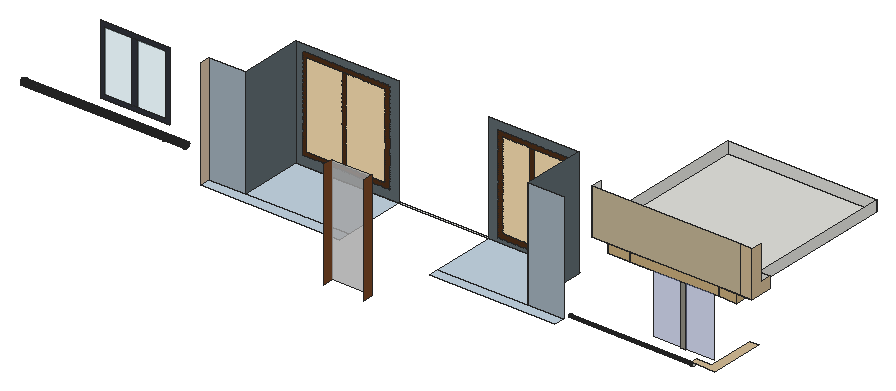
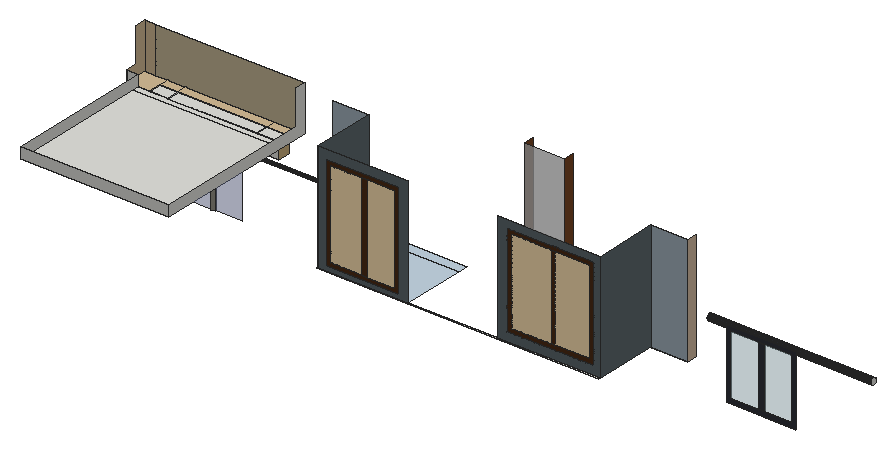
# SketchUp Ruby script. Lengths in inches.
U = 1.inch
M = Sketchup.active_model
def pt(a) = Geom::Point3d.new(a.map { |v| v * U })
def face(e, loops, mat)
  f = e.add_face(loops[0].map { |a| pt(a) })
  loops[1..].each { |l| e.add_face(l.map { |a| pt(a) }).erase! }
  f.material = f.back_material = mat if mat
  f
end
# faces: each face lists its corners as indices into pts; further lists are holes
def faces(e, pts, list, mat = nil) = list.each { |f| face(e, (f[0].is_a?(Array) ? f : [f]).map { |l| l.map { |i| pts[i] } }, mat) }
# xy, xz, yz: faces in a plane at the given z, y or x. An outline is a flat list of corners, or four numbers for a rectangle; further outlines are holes
def ring(l) = l.size == 4 ? [[l[0], l[1]], [l[2], l[1]], [l[2], l[3]], [l[0], l[3]]] : l.each_slice(2).to_a
def flat(e, list, mat, &to3) = list.each { |f| face(e, (f[0].is_a?(Array) ? f : [f]).map { |l| ring(l).map { |u, v| to3.(u, v) } }, mat) }
def xy(e, z, list, mat = nil) = flat(e, list, mat) { |x, y| [x, y, z] }
def xz(e, y, list, mat = nil) = flat(e, list, mat) { |x, z| [x, y, z] }
def yz(e, x, list, mat = nil) = flat(e, list, mat) { |y, z| [x, y, z] }
def lines(e, pts, list) = list.each { |a, b| e.add_line(pt(pts[a]), pt(pts[b])) }
# prism: a flat outline (further loops are holes) pulled along v
def prism(e, loops, v, mat = nil)
  f = face(e, loops, mat); d = Geom::Vector3d.new(v.map { |x| x * U })
  f.pushpull(f.normal.samedirection?(d) ? d.length : -d.length)
end
def box(e, o, s, mat = nil) = prism(e, [[o, [o[0] + s[0], o[1], o[2]], [o[0] + s[0], o[1] + s[1], o[2]], [o[0], o[1] + s[1], o[2]]]], [0, 0, s[2]], mat)
def at(x, y, z, deg = 0) = Geom::Transformation.translation(pt([x, y, z])) * Geom::Transformation.rotation(ORIGIN, Z_AXIS, deg.degrees)
def axes(o, x, y, z) = Geom::Transformation.new([*x, 0, *y, 0, *z, 0, *pt(o).to_a, 1])
def part(name) = M.definitions.add(name)
# library, detail: a bought-in or finely detailed component or shape, given as its bounding box
def library(name, o, s) = part(name).tap { |d| box(d.entities, o, s) }
def detail(e, o, s) = box(e.add_group.entities, o, s)
def put(e, d, t, mat = nil) = e.add_instance(d, t).tap { |i| i.material = mat if mat }
def group(e, t, mat = nil) = e.add_group.tap { |g| g.transformation = t; g.material = mat if mat }.entities
root = M.entities
M.materials.add("[0032_Moccasin]").color = [255, 228, 181]
M.materials.add("[Formica Beige]").color = [211, 187, 149]
M.materials.add("[Formica Graystone]").color = [149, 146, 135]
M.materials.add("[Formica Laminate Dark]").color = [50, 53, 60]
M.materials.add("[Formica Laminate Light]").color = [213, 189, 164]
M.materials.add("[Formica Speckled Grey]").color = [94, 105, 111]
M.materials.add("[Quartz Light Brown]").color = [199, 184, 152]
M.materials.add("[Terrazzo Light Blue]1").color = [165, 180, 191]
M.materials.add("[Terrazzo Light Blue]2").color = [196, 214, 227]
M.materials.add("[Translucent Glass Safety]").color = [204, 235, 244]
M.materials["[Translucent Glass Safety]"].alpha = 0.5
M.materials.add("[Translucent Glass Sky Reflection]").color = [126, 138, 183]
M.materials["[Translucent Glass Sky Reflection]"].alpha = 0.52
M.materials.add("[Translucent Resin Crush Gray]").color = [201, 201, 201]
M.materials["[Translucent Resin Crush Gray]"].alpha = 0.8
M.materials.add("[Wood Floor Light]").color = [204, 176, 127]
M.materials.add("[Wood Veneer 01]").color = [79, 46, 24]
M.materials.add("[Wood Veneer 01]2").color = [120, 70, 37]
xy(root,525,[[238.58,216.84,549.2,218.65]])
xy(root,525,[[198.57,135.71,351.88,147.05],[450.54,135.71,588.3,147.05],[238.58,147.05,351.88,216.84],[450.54,147.05,549.2,216.84]],"[Terrazzo Light Blue]2")
xy(root,544.8125,[[666.73,124.73,667.14,124.78,667.51,124.94,667.84,125.1875,668.09,125.51,668.24,125.89,668.3,126.29,668.24,126.7,668.09,127.07,667.84,127.4,667.51,127.65,667.14,127.8,666.73,127.86,666.33,127.8,665.95,127.65,665.63,127.4,665.38,127.07,665.22,126.7,665.17,126.29,665.22,125.89,665.38,125.51,665.63,125.1875,665.95,124.94,666.33,124.78],[693.42,124.73,693.83,124.78,694.2,124.94,694.53,125.1875,694.77,125.51,694.93,125.89,694.98,126.29,694.93,126.7,694.77,127.07,694.53,127.4,694.2,127.65,693.83,127.8,693.42,127.86,693.02,127.8,692.64,127.65,692.32,127.4,692.07,127.07,691.91,126.7,691.86,126.29,691.91,125.89,692.07,125.51,692.32,125.1875,692.64,124.94,693.02,124.78],[709.48,124.73,709.89,124.78,710.26,124.94,710.59,125.1875,710.84,125.51,710.99,125.89,711.05,126.29,710.99,126.7,710.84,127.07,710.59,127.4,710.26,127.65,709.89,127.8,709.48,127.86,709.08,127.8,708.7,127.65,708.38,127.4,708.13,127.07,707.97,126.7,707.92,126.29,707.97,125.89,708.13,125.51,708.38,125.1875,708.7,124.94,709.08,124.78]])
xy(root,545.4375,[[621.3,124.73,621.7,124.78,622.08,124.94,622.3125,125.12,620.28,125.12,620.51,124.94,620.89,124.78],[634.92,124.73,635.33,124.78,635.7,124.94,635.9375,125.12,636.03,125.1875,636.27,125.51,636.43,125.89,636.48,126.29,636.43,126.7,636.27,127.07,636.03,127.4,635.7,127.65,635.33,127.8,634.92,127.86,634.52,127.8,634.14,127.65,633.82,127.4,633.57,127.07,633.41,126.7,633.36,126.29,633.41,125.89,633.57,125.51,633.82,125.1875,633.91,125.12,634.14,124.94,634.52,124.78],[651.73,124.73,652.14,124.78,652.51,124.94,652.75,125.12,650.72,125.12,650.95,124.94,651.33,124.78],[735.61,124.73,736.01,124.78,736.39,124.94,736.625,125.12,736.71,125.1875,736.96,125.51,737.12,125.89,737.17,126.29,737.12,126.7,736.96,127.07,736.71,127.4,736.39,127.65,736.01,127.8,735.61,127.86,735.2,127.8,734.83,127.65,734.5,127.4,734.26,127.07,734.1,126.7,734.05,126.29,734.1,125.89,734.26,125.51,734.5,125.1875,734.83,124.94,735.2,124.78],[620.28,125.12,622.3125,125.12,622.4,125.1875,622.65,125.51,622.81,125.89,622.86,126.29,622.81,126.7,622.65,127.07,622.4,127.4,622.08,127.65,621.7,127.8,621.3,127.86,620.89,127.8,620.51,127.65,620.19,127.4,619.94,127.07,619.79,126.7,619.73,126.29,619.79,125.89,619.94,125.51,620.19,125.1875],
  [650.72,125.12,652.75,125.12,652.84,125.1875,653.09,125.51,653.24,125.89,653.3,126.29,653.24,126.7,653.09,127.07,652.84,127.4,652.51,127.65,652.14,127.8,651.73,127.86,651.33,127.8,650.95,127.65,650.63,127.4,650.38,127.07,650.22,126.7,650.17,126.29,650.22,125.89,650.38,125.51,650.63,125.1875]])
xy(root,545.78,[[680.8,124.73,681.2,124.78,681.58,124.94,681.9,125.1875,681.96,125.26,679.63,125.26,679.69,125.1875,680.01,124.94,680.39,124.78],[722.42,124.73,722.83,124.78,723.2,124.94,723.53,125.1875,723.58,125.26,721.26,125.26,721.32,125.1875,721.64,124.94,722.02,124.78],[679.63,125.26,681.96,125.26,682.15,125.51,682.31,125.89,682.36,126.29,682.31,126.7,682.15,127.07,681.9,127.4,681.58,127.65,681.32,127.75,680.27,127.75,680.01,127.65,679.69,127.4,679.44,127.07,679.29,126.7,679.23,126.29,679.29,125.89,679.44,125.51],[721.26,125.26,723.58,125.26,723.77,125.51,723.93,125.89,723.98,126.29,723.93,126.7,723.77,127.07,723.53,127.4,723.2,127.65,722.95,127.75,721.9,127.75,721.64,127.65,721.32,127.4,721.07,127.07,720.91,126.7,720.86,126.29,720.91,125.89,721.07,125.51],[680.27,127.75,681.32,127.75,681.2,127.8,680.8,127.86,680.39,127.8],
  [721.9,127.75,722.95,127.75,722.83,127.8,722.42,127.86,722.02,127.8]])
xy(root,549,[[748.22,122.79,774.15,122.79,774.15,182.57,764.59,182.57,764.59,130.07,748.22,130.07]],"[Formica Beige]")
xy(root,560.5625,[[165.13,126.7,165.6,126.76,166.03,126.95,166.41,127.23,166.7,127.61,166.88,128.05,166.89,128.15,166.94,128.51,166.88,128.98,166.7,129.42,166.41,129.8,166.03,130.08,165.6,130.27,165.13,130.33,164.66,130.27,164.22,130.08,163.85,129.8,163.56,129.42,163.375,128.98,163.31,128.51,163.36,128.15,163.375,128.05,163.56,127.61,163.85,127.23,164.22,126.95,164.66,126.76]])
xy(root,561.5,[[110.19,126.7,110.66,126.76,111.1,126.95,111.47,127.23,111.76,127.61,111.94,128.05,112,128.51,111.94,128.98,111.76,129.42,111.47,129.8,111.1,130.08,110.66,130.27,110.19,130.33,109.72,130.27,109.28,130.08,108.91,129.8,108.62,129.42,108.4375,128.98,108.38,128.51,108.4375,128.05,108.62,127.61,108.91,127.23,109.28,126.95,109.72,126.76]])
xy(root,561.8125,[[131.69,126.7,132.16,126.76,132.6,126.95,132.97,127.23,133.26,127.61,133.44,128.05,133.5,128.51,133.44,128.98,133.26,129.42,132.97,129.8,132.6,130.08,132.16,130.27,131.69,130.33,131.22,130.27,130.78,130.08,130.41,129.8,130.12,129.42,129.9375,128.98,129.88,128.51,129.9375,128.05,130.12,127.61,130.41,127.23,130.78,126.95,131.22,126.76]])
xy(root,562.6875,[[75.69,126.7,76.16,126.76,76.6,126.95,76.97,127.23,77.26,127.61,77.44,128.05,77.5,128.51,77.44,128.98,77.26,129.42,76.97,129.8,76.6,130.08,76.16,130.27,75.69,130.33,75.22,130.27,74.78,130.08,74.41,129.8,74.12,129.42,73.9375,128.98,73.88,128.51,73.9375,128.05,74.12,127.61,74.41,127.23,74.78,126.95,75.22,126.76]])
xy(root,562.9375,[[60.69,126.7,61.16,126.76,61.6,126.95,61.97,127.23,62.26,127.61,62.44,128.05,62.5,128.51,62.44,128.98,62.26,129.42,61.97,129.8,61.6,130.08,61.16,130.27,60.69,130.33,60.22,130.27,59.78,130.08,59.41,129.8,59.12,129.42,58.9375,128.98,58.88,128.51,58.9375,128.05,59.12,127.61,59.41,127.23,59.78,126.95,60.22,126.76]])
xy(root,564.0625,[[29.13,126.7,29.6,126.76,30.03,126.95,30.41,127.23,30.7,127.61,30.88,128.05,30.94,128.51,30.88,128.98,30.7,129.42,30.41,129.8,30.03,130.08,29.6,130.27,29.13,130.33,28.66,130.27,28.22,130.08,27.85,129.8,27.56,129.42,27.375,128.98,27.31,128.51,27.375,128.05,27.56,127.61,27.85,127.23,28.22,126.95,28.66,126.76]])
xy(root,564.5625,[[44.81,126.7,45.28,126.76,45.72,126.95,46.1,127.23,46.38,127.61,46.57,128.05,46.63,128.51,46.57,128.98,46.38,129.42,46.1,129.8,45.72,130.08,45.28,130.27,44.81,130.33,44.35,130.27,43.91,130.08,43.53,129.8,43.25,129.42,43.0625,128.98,43,128.51,43.0625,128.05,43.25,127.61,43.53,127.23,43.91,126.95,44.35,126.76]])
xy(root,564.65,[[16.13,126.7,16.6,126.76,17.03,126.95,17.41,127.23,17.7,127.61,17.88,128.05,17.94,128.51,17.88,128.98,17.7,129.42,17.41,129.8,17.03,130.08,16.6,130.27,16.13,130.33,15.66,130.27,15.22,130.08,14.85,129.8,14.56,129.42,14.375,128.98,14.31,128.51,14.375,128.05,14.56,127.61,14.85,127.23,15.22,126.95,15.66,126.76],[181.81,126.7,182.28,126.76,182.72,126.95,183.1,127.23,183.38,127.61,183.57,128.05,183.63,128.51,183.57,128.98,183.38,129.42,183.1,129.8,182.72,130.08,182.28,130.27,181.81,130.33,181.35,130.27,180.91,130.08,180.53,129.8,180.25,129.42,180.0625,128.98,180,128.51,180.0625,128.05,180.25,127.61,180.53,127.23,180.91,126.95,181.35,126.76]])
xy(root,565.4375,[[149.06,126.7,149.53,126.76,149.97,126.95,150.35,127.23,150.63,127.61,150.82,128.05,150.88,128.51,150.82,128.98,150.63,129.42,150.35,129.8,149.97,130.08,149.53,130.27,149.06,130.33,148.6,130.27,148.16,130.08,147.78,129.8,147.5,129.42,147.3125,128.98,147.25,128.51,147.3125,128.05,147.5,127.61,147.78,127.23,148.16,126.95,148.6,126.76]])
xy(root,566.11,[[89.81,126.7,90.28,126.76,90.72,126.95,91.1,127.23,91.38,127.61,91.57,128.05,91.63,128.51,91.57,128.98,91.38,129.42,91.1,129.8,90.72,130.08,90.28,130.27,89.81,130.33,89.35,130.27,88.91,130.08,88.53,129.8,88.25,129.42,88.0625,128.98,88,128.51,88.0625,128.05,88.25,127.61,88.53,127.23,88.91,126.95,89.35,126.76]])
xy(root,591.38,[[619.29,168.64,644.11,182.57],[741.11,168.64,761.42,182.57]])
xy(root,591.38,[[644.11,168.64,741.11,182.57]],"[Wood Floor Light]")
xy(root,609,[[619.29,168.64,644.11,182.57],[644.11,168.64,741.11,182.57],[741.11,168.64,761.42,182.57],[611.125,182.57,774.15,189.24],[611.125,189.24,774.15,344.36]])
xy(root,609,[[611.125,157.7,619.29,182.57],[619.29,157.7,644.11,168.64],[644.11,157.7,741.11,168.64],[741.11,157.7,761.42,168.64],[761.42,157.7,786.87,182.57]],"[Formica Beige]")
xz(root,88.2,[[380.3,515.72,424.94,634.57]],"[Translucent Resin Crush Gray]")
xz(root,147.05,[[198.57,525,238.58,645],[549.2,525,588.3,645]],"[Terrazzo Light Blue]1")
xz(root,157.7,[[774.15,609,786.87,658.875]],"[Formica Beige]")
xz(root,157.7,[[611.125,609,774.15,658.875]],"[Quartz Light Brown]")
xz(root,168.64,[[619.29,591.38,644.11,609],[644.11,591.38,741.11,609],[741.11,591.38,761.42,609]],"[Wood Floor Light]")
xz(root,182.57,[[619.29,591.38,644.11,609],[644.11,591.38,741.11,609],[741.11,591.38,761.42,609],[774.15,609,786.87,621]])
xz(root,182.57,[[689.22,516.23,694.06,582.39]],"[Formica Graystone]")
xz(root,182.57,[[659.44,516.23,689.22,582.39],[694.06,516.23,725.6,582.39]],"[Translucent Glass Sky Reflection]")
xz(root,191.15,[[[43.9375,531.79,120.375,608.22],[48.9,536.75,115.4,603.25]],[78.96,536.75,85.19,603.25]],"[Formica Laminate Dark]")
xz(root,191.15,[[48.9,536.75,78.96,603.25],[85.19,536.75,115.4,603.25]],"[Translucent Glass Safety]")
xz(root,216.84,[[465.16,534.55,494.11,630.15],[501.07,534.55,535.45,630.15],[250.54,539.68,288.48,632.46],[293.68,539.68,336.57,632.46]],"[0032_Moccasin]")
xz(root,216.84,[[[238.58,525,351.88,645],[245.71,534.85,341.39,637.29]],[[450.54,525,549.2,645],[459.93,529.32,540.68,635.38]]],"[Formica Speckled Grey]")
xz(root,216.84,[[[459.93,529.32,540.68,635.38],[465.16,534.55,535.45,630.15]],[494.11,534.55,501.07,630.15],[[245.71,534.85,341.39,637.29],[250.54,539.68,336.57,632.46]],[288.48,539.68,293.68,632.46]],"[Wood Veneer 01]")
xz(root,344.36,[[611.125,609,774.15,621]])
yz(root,9,[[128.15,560.5625,127.31,560.67,126.52,561,125.85,561.51,125.33,562.1875,125.01,562.97,124.9,563.8125,125.01,564.65,125.33,565.4375,125.85,566.11,126.52,566.625,127.31,566.95,128.15,567.0625,128.99,566.95,129.77,566.625,130.45,566.11,130.96,565.4375,131.29,564.65,131.4,563.8125,131.29,562.97,130.96,562.1875,130.45,561.51,129.77,561,128.99,560.67]])
yz(root,198.57,[[135.71,525,147.05,645]],"[Formica Laminate Light]")
yz(root,238.58,[[147.05,525,216.84,645]],"[Formica Speckled Grey]")
yz(root,380.3,[[77.26,515.72,88.2,634.57]],"[Wood Veneer 01]2")
yz(root,424.94,[[77.26,515.72,88.2,634.57]],"[Wood Veneer 01]2")
yz(root,549.2,[[147.05,525,216.84,645]],"[Formica Speckled Grey]")
yz(root,611.125,[[157.7,609,344.36,609,344.36,621,169.39,621,169.39,658.875,157.7,658.875]])
yz(root,619.29,[[168.64,591.38,182.57,609]],"[Wood Floor Light]")
yz(root,644.11,[[168.64,591.38,182.57,609]])
yz(root,741.11,[[168.64,591.38,182.57,609]])
yz(root,748.22,[[126.51,543.63,126.88,543.68,127.23,543.82,127.52,544.05,127.75,544.35,127.9,544.69,127.95,545.07,127.9,545.4375,127.75,545.78,127.52,546.08,127.23,546.31,126.88,546.45,126.51,546.5,126.14,546.45,125.79,546.31,125.49,546.08,125.26,545.78,125.12,545.4375,125.07,545.07,125.12,544.69,125.26,544.35,125.49,544.05,125.79,543.82,126.14,543.68]])
yz(root,761.42,[[168.64,591.38,182.57,609]],"[Wood Floor Light]")
yz(root,774.15,[[182.57,609,344.36,621]])
yz(root,786.87,[[157.7,609,182.57,609,182.57,621,169.39,621,169.39,658.875,157.7,658.875]],"[Formica Beige]")
p = [[748.22,126.51,543.63],[748.22,126.14,543.68],[611.125,126.14,543.68],[611.125,126.51,543.63],[748.22,126.88,543.68],[611.125,126.88,543.68],
  [748.22,125.79,543.82],[611.125,125.79,543.82],[748.22,127.23,543.82],[611.125,127.23,543.82],[748.22,125.49,544.05],[611.125,125.49,544.05],
  [748.22,127.52,544.05],[611.125,127.52,544.05],[748.22,125.26,544.35],[611.125,125.26,544.35],[748.22,127.75,544.35],[611.125,127.75,544.35],
  [748.22,125.12,544.69],[611.125,125.12,544.69],[748.22,127.9,544.69],[611.125,127.9,544.69],[748.22,125.07,545.07],[611.125,125.07,545.07],
  [748.22,127.95,545.07],[611.125,127.95,545.07],[748.22,125.12,545.4375],[736.625,125.12,545.4375],[734.59,125.12,545.4375],[652.75,125.12,545.4375],
  [650.72,125.12,545.4375],[635.9375,125.12,545.4375],[633.91,125.12,545.4375],[622.3125,125.12,545.4375],[620.28,125.12,545.4375],[611.125,125.12,545.4375],
  [748.22,127.9,545.4375],[611.125,127.9,545.4375],[748.22,125.26,545.78],[723.58,125.26,545.78],[721.26,125.26,545.78],[681.96,125.26,545.78],
  [679.63,125.26,545.78],[611.125,125.26,545.78],[748.22,127.75,545.78],[611.125,127.75,545.78],[680.27,127.75,545.78],[681.32,127.75,545.78],
  [721.9,127.75,545.78],[722.95,127.75,545.78],[748.22,125.49,546.08],[611.125,125.49,546.08],[748.22,127.52,546.08],[611.125,127.52,546.08],
  [748.22,125.79,546.31],[611.125,125.79,546.31],[748.22,127.23,546.31],[611.125,127.23,546.31],[748.22,126.14,546.45],[611.125,126.14,546.45],
  [748.22,126.88,546.45],[611.125,126.88,546.45],[748.22,126.51,546.5],[611.125,126.51,546.5],[9,127.31,560.67],[9,128.15,560.5625],
  [163.36,128.15,560.5625],[166.89,128.15,560.5625],[189.57,128.15,560.5625],[189.57,127.31,560.67],[9,128.99,560.67],[189.57,128.99,560.67],
  [9,126.52,561],[189.57,126.52,561],[9,129.77,561],[189.57,129.77,561],[9,125.85,561.51],[189.57,125.85,561.51],
  [9,130.45,561.51],[189.57,130.45,561.51],[9,125.33,562.1875],[189.57,125.33,562.1875],[9,130.96,562.1875],[189.57,130.96,562.1875],
  [9,125.01,562.97],[189.57,125.01,562.97],[9,131.29,562.97],[189.57,131.29,562.97],[9,124.9,563.8125],[189.57,124.9,563.8125],
  [9,131.4,563.8125],[189.57,131.4,563.8125],[9,125.01,564.65],[189.57,125.01,564.65],[9,131.29,564.65],[189.57,131.29,564.65],
  [9,125.33,565.4375],[189.57,125.33,565.4375],[9,130.96,565.4375],[189.57,130.96,565.4375],[9,125.85,566.11],[189.57,125.85,566.11],
  [9,130.45,566.11],[189.57,130.45,566.11],[9,126.52,566.625],[189.57,126.52,566.625],[9,129.77,566.625],[189.57,129.77,566.625],
  [9,127.31,566.95],[189.57,127.31,566.95],[9,128.99,566.95],[189.57,128.99,566.95],[9,128.15,567.0625],[189.57,128.15,567.0625]]
faces(root,p,[[0,1,2,3],[4,0,3,5],[1,6,7,2],[8,4,5,9],[6,10,11,7],[12,8,9,13],[10,14,15,11],[16,12,13,17],
  [14,18,19,15],[20,16,17,21],[18,22,23,19],[24,20,21,25],[22,26,27,28,29,30,31,32,33,34,35,23],[36,24,25,37],[26,38,39,40,41,42,43,35,34,33,32,31,30,29,28,27],[44,36,37,45,46,47,48,49],
  [38,50,51,43,42,41,40,39],[52,44,49,48,47,46,45,53],[50,54,55,51],[56,52,53,57],[54,58,59,55],[60,56,57,61],[58,62,63,59],[62,60,61,63],
  [64,65,66,67,68,69],[65,70,71,68,67,66],[72,64,69,73],[70,74,75,71],[76,72,73,77],[74,78,79,75],[80,76,77,81],[78,82,83,79],
  [84,80,81,85],[82,86,87,83],[88,84,85,89],[86,90,91,87],[92,88,89,93],[90,94,95,91],[96,92,93,97],[94,98,99,95],
  [100,96,97,101],[98,102,103,99],[104,100,101,105],[102,106,107,103],[108,104,105,109],[106,110,111,107],[112,108,109,113],[110,112,113,111]],"[Formica Laminate Dark]")
